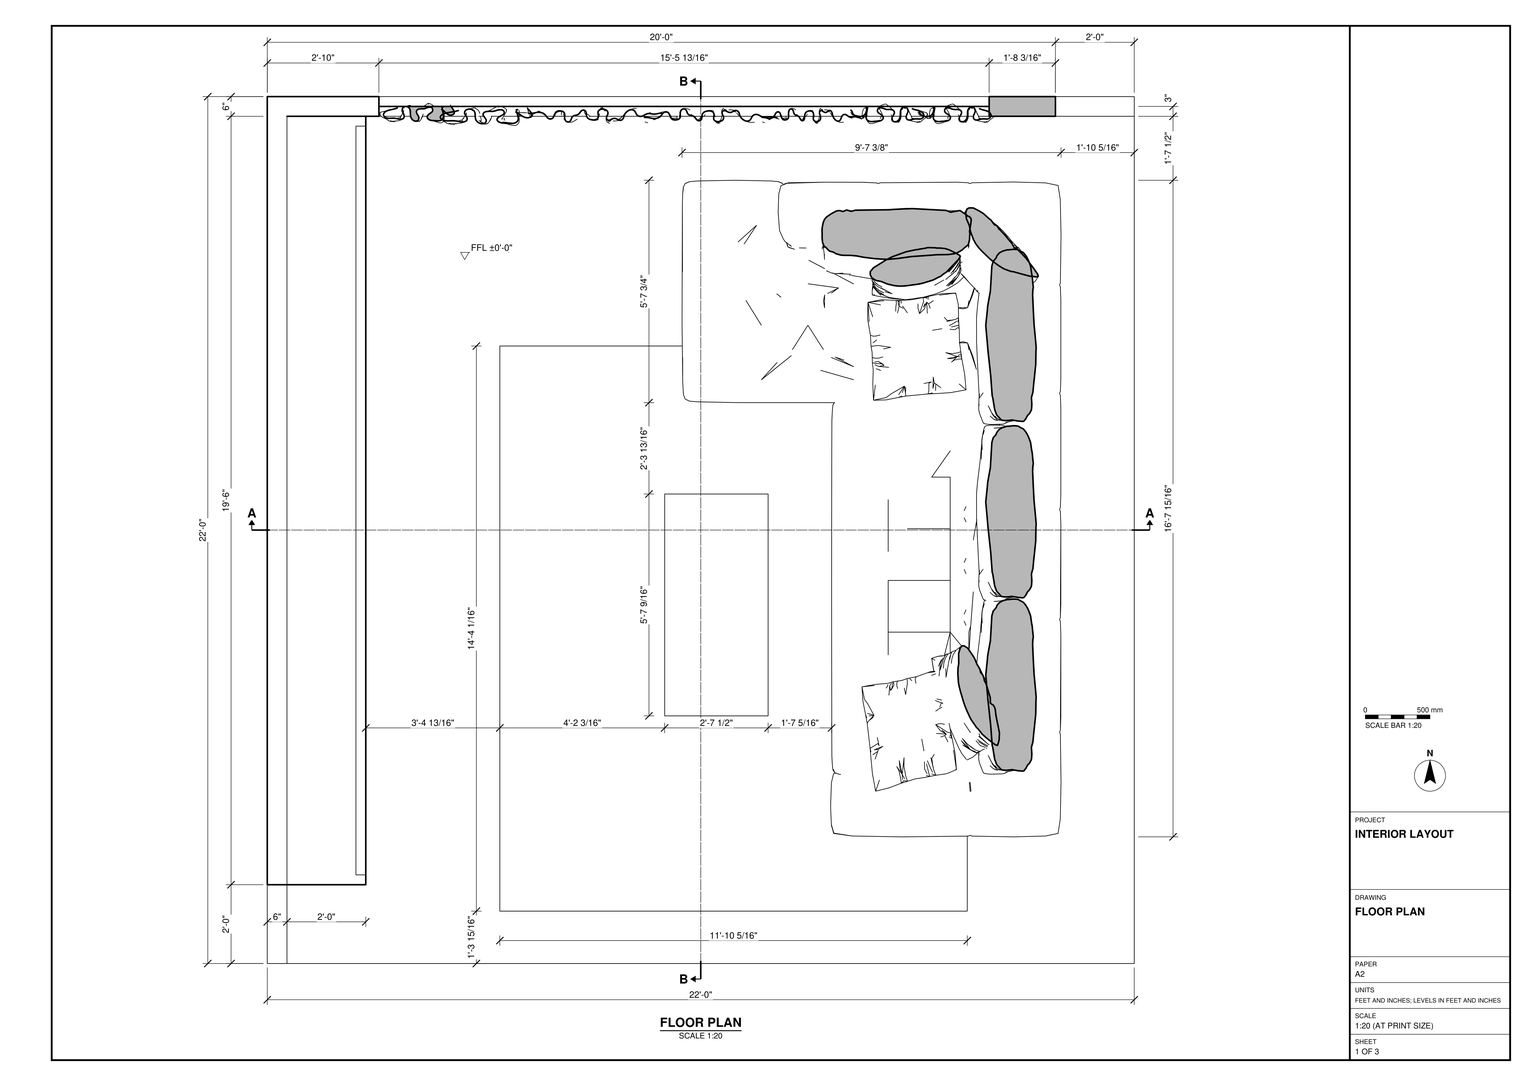
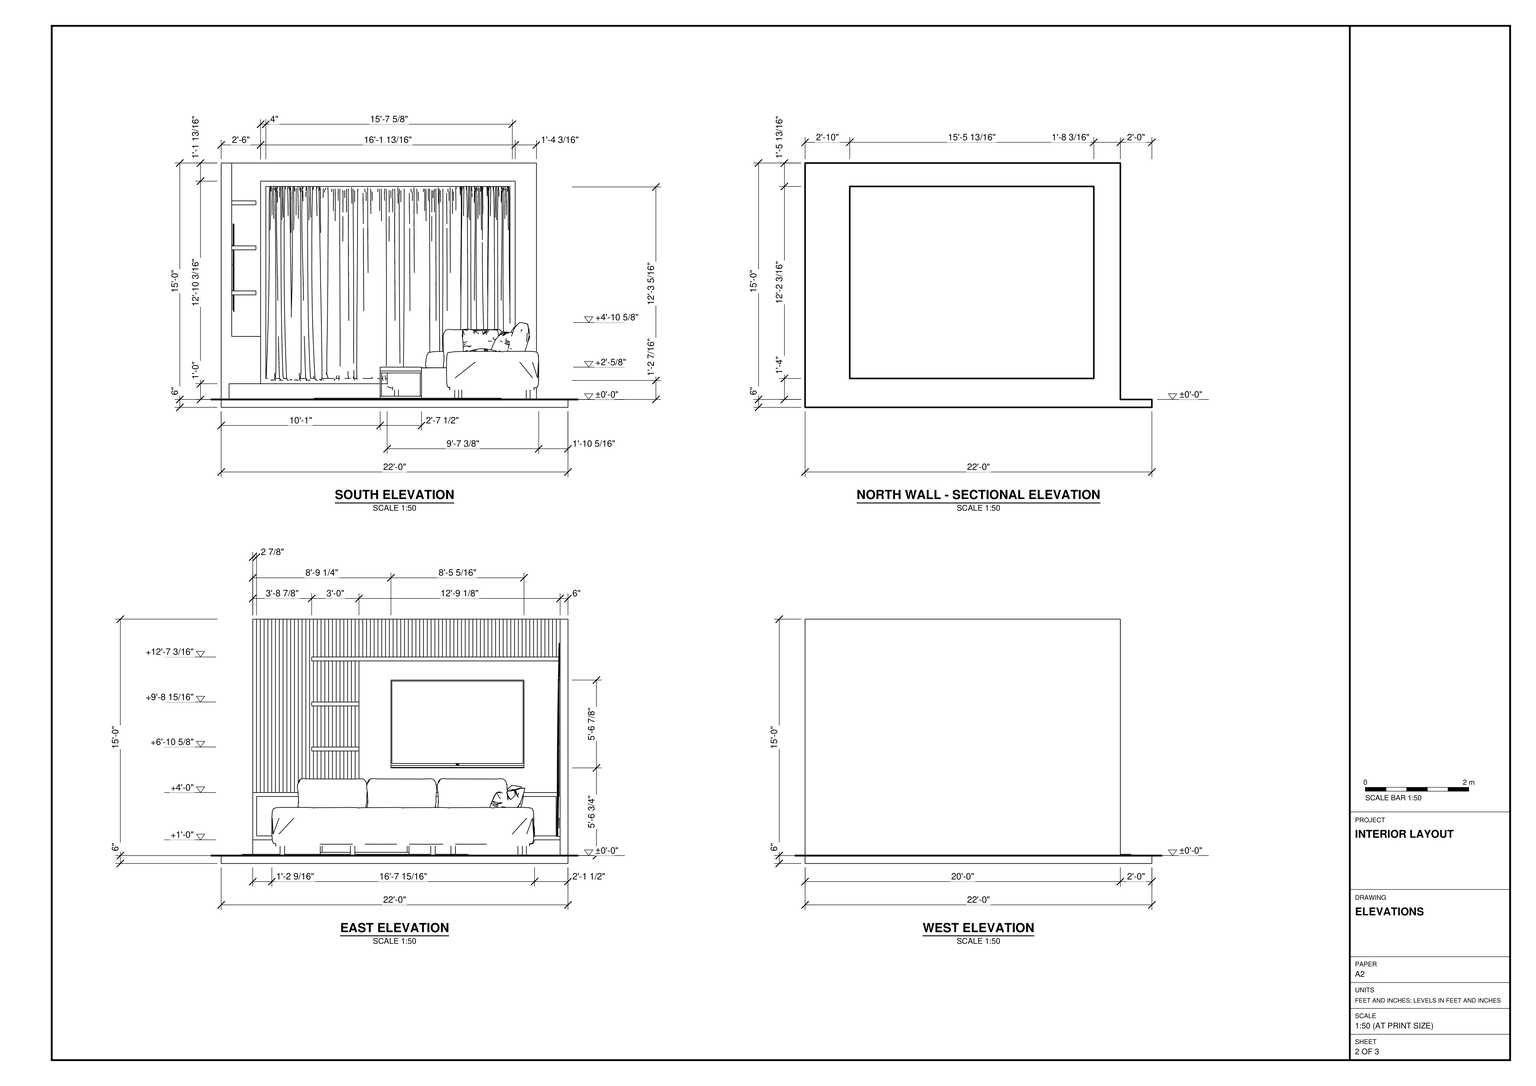
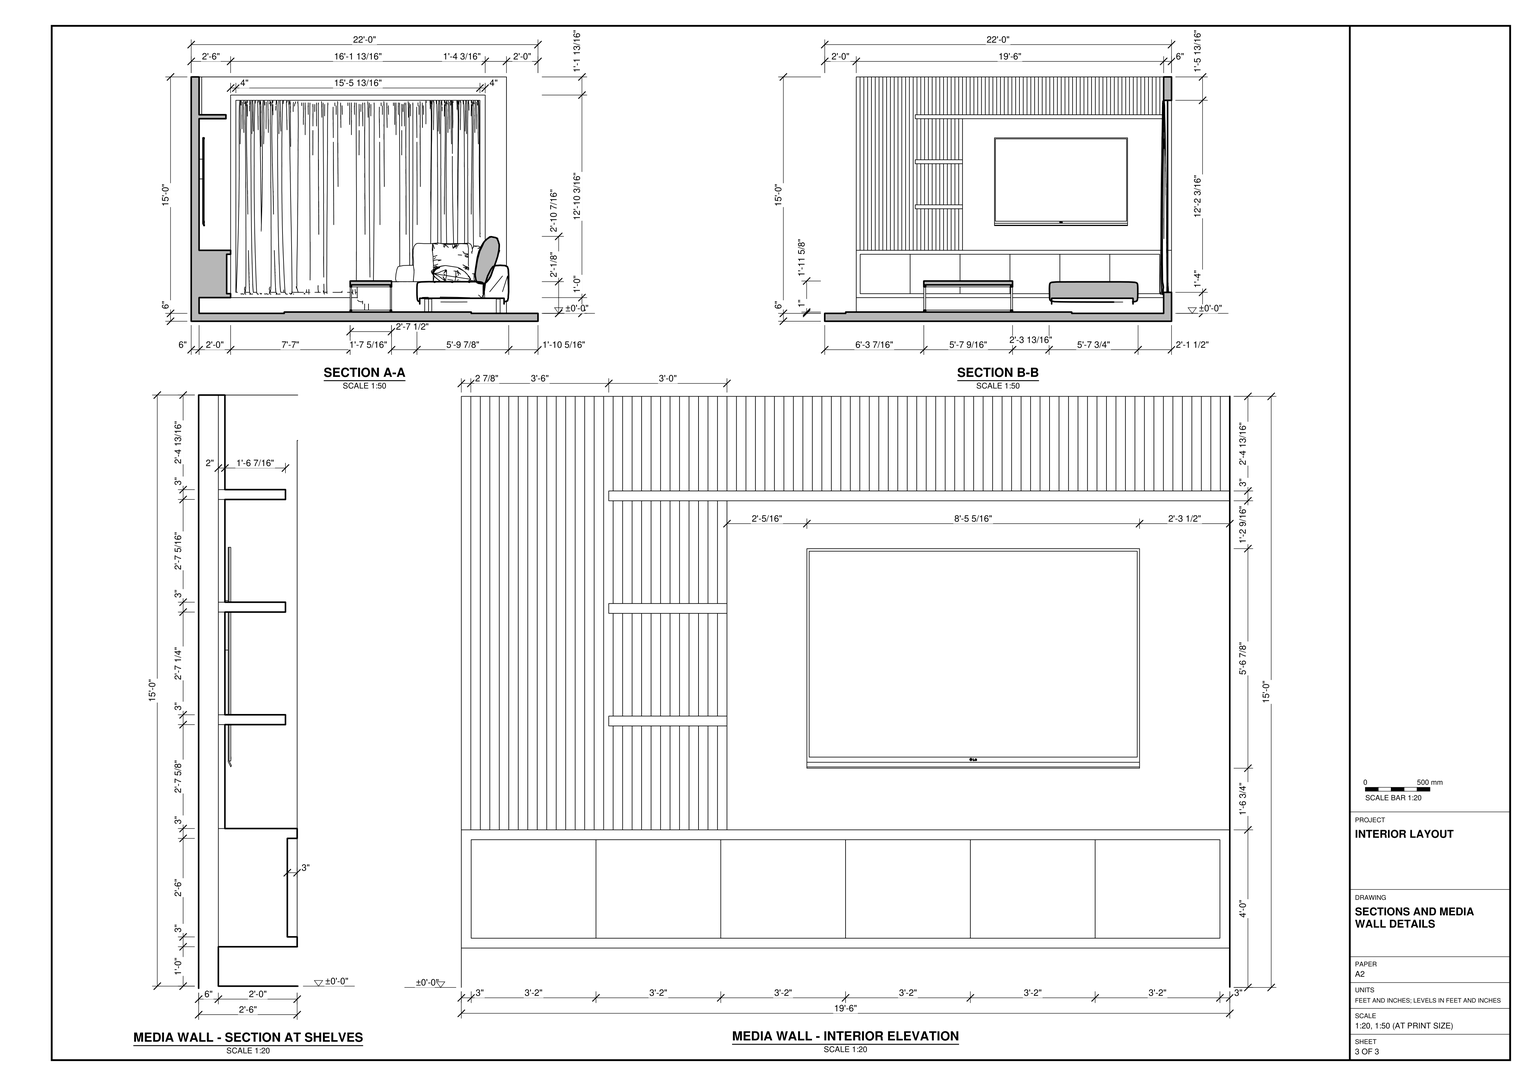
Build the living room in SketchUp from task_files/diagram_01.pdf. Work in feet and inches. The overall model is 22'-0" wide, 22'-0" deep and 15'-6" high. Set the finished floor at ±0'-0", with the 6" slab below it. Use the floor plan to place the 6" walls along the north and west sides, leaving the other sides open as drawn. Form the wide opening in the north wall, retaining the sill, head and unequal side returns. Hang the curtains across the opening.

Use the media wall elevation and shelf section to build the joinery on the inside face of the west wall. Include the raised cabinet with divided fronts, the vertical slats, the long upper shelf and the two shorter shelves beside the television. Place the sectional sofa opposite the television, with its long back on the east side and its chaise extending west at the north end. Set the low rectangular table between the sofa and cabinet, on the rug shown in plan. Decor and loose items, including the rug, cushions and television, may be any suitable library components.

Keep the walls, slab and each furniture or joinery piece in separate groups or components, and use components for repeated parts. Save one SketchUp model as output_files/living_room_with_a_built_in_media_wall.skp.

# SketchUp Ruby script. Lengths in inches.
U = 1.inch
M = Sketchup.active_model
def pt(a) = Geom::Point3d.new(a.map { |v| v * U })
def face(e, loops, mat)
  f = e.add_face(loops[0].map { |a| pt(a) })
  loops[1..].each { |l| e.add_face(l.map { |a| pt(a) }).erase! }
  f.material = f.back_material = mat if mat
  f
end
# faces: each face lists its corners as indices into pts; further lists are holes
def faces(e, pts, list, mat = nil) = list.each { |f| face(e, (f[0].is_a?(Array) ? f : [f]).map { |l| l.map { |i| pts[i] } }, mat) }
# xy, xz, yz: faces in a plane at the given z, y or x. An outline is a flat list of corners, or four numbers for a rectangle; further outlines are holes
def ring(l) = l.size == 4 ? [[l[0], l[1]], [l[2], l[1]], [l[2], l[3]], [l[0], l[3]]] : l.each_slice(2).to_a
def flat(e, list, mat, &to3) = list.each { |f| face(e, (f[0].is_a?(Array) ? f : [f]).map { |l| ring(l).map { |u, v| to3.(u, v) } }, mat) }
def xy(e, z, list, mat = nil) = flat(e, list, mat) { |x, y| [x, y, z] }
def xz(e, y, list, mat = nil) = flat(e, list, mat) { |x, z| [x, y, z] }
def yz(e, x, list, mat = nil) = flat(e, list, mat) { |y, z| [x, y, z] }
def lines(e, pts, list) = list.each { |a, b| e.add_line(pt(pts[a]), pt(pts[b])) }
# prism: a flat outline (further loops are holes) pulled along v
def prism(e, loops, v, mat = nil)
  f = face(e, loops, mat); d = Geom::Vector3d.new(v.map { |x| x * U })
  f.pushpull(f.normal.samedirection?(d) ? d.length : -d.length)
end
def box(e, o, s, mat = nil) = prism(e, [[o, [o[0] + s[0], o[1], o[2]], [o[0] + s[0], o[1] + s[1], o[2]], [o[0], o[1] + s[1], o[2]]]], [0, 0, s[2]], mat)
def at(x, y, z, deg = 0) = Geom::Transformation.translation(pt([x, y, z])) * Geom::Transformation.rotation(ORIGIN, Z_AXIS, deg.degrees)
def axes(o, x, y, z) = Geom::Transformation.new([*x, 0, *y, 0, *z, 0, *pt(o).to_a, 1])
def part(name) = M.definitions.add(name)
# library, detail: a bought-in or finely detailed component or shape, given as its bounding box
def library(name, o, s) = part(name).tap { |d| box(d.entities, o, s) }
def detail(e, o, s) = box(e.add_group.entities, o, s)
def put(e, d, t, mat = nil) = e.add_instance(d, t).tap { |i| i.material = mat if mat }
def group(e, t, mat = nil) = e.add_group.tap { |g| g.transformation = t; g.material = mat if mat }.entities
root = M.entities
M.materials.add("DefaultMaterial~1").color = [7, 7, 6]
M.materials.add("[0131_Silver]").color = [192, 192, 192]
M.materials.add("[0136_Charcoal]").color = [35, 35, 35]
M.materials.add("[Color_008]3").color = [29, 29, 29]
M.materials.add("[Formica Graystone]").color = [188, 184, 170]
M.materials.add("[Translucent Glass Blue]").color = [100, 149, 237]
M.materials["[Translucent Glass Blue]"].alpha = 0.5
c1 = library("TV (1)",[0,0,0],[57.09,0.98,33.46])
c2 = library("sofa (1)",[21.72,74.94,0],[120.18,81.27,34.35])
c3 = part("Group\#116")
box(c3.entities,[0,0,0],[0.98,0.98,11.8125])
c4 = part("center table rec")
g1 = group(c4.entities,at(39.79,0,0,90))
g2 = group(g1,at(0,0,0),"[Color_008]3")
put(g2,c3,at(0,-7.46,0.98))
g3 = group(g2,at(0,38.8,0.98))
box(g3,[0,0,0],[0.98,0.98,11.8125])
g4 = group(g2,at(30.51,38.8,0.98))
box(g4,[0,0,0],[0.98,0.98,11.8125])
put(g2,c3,at(30.51,-7.46,0.98))
g5 = group(g2,at(0,0,12.8))
prism(g5,[[[31.5,-7.46,0],[0,-7.46,0],[0,39.79,0],[31.5,39.79,0]],[[30.51,-6.47,0],[30.51,38.8,0],[0.98,38.8,0],[0.98,-6.47,0]]],[0,0,0.98])
g6 = group(g2,at(0,0,0))
prism(g6,[[[31.5,-7.46,0],[0,-7.46,0],[0,39.79,0],[31.5,39.79,0]],[[30.51,-6.47,0],[30.51,38.8,0],[0.98,38.8,0],[0.98,-6.47,0]]],[0,0,0.98])
g7 = group(g1,at(0,0,13.78))
xy(g7,0,[[0,-7.46,31.5,39.79]],"DefaultMaterial~1")
xy(g7,1.97,[[0.06,-7.4,0.08,-7.38,0.08,39.71,0.06,39.73],[0.06,-7.4,31.4375,-7.4,31.42,-7.38,0.08,-7.38],[31.4375,-7.4,31.4375,39.73,31.42,39.71,31.42,-7.38],[0.08,-7.38,31.42,39.71],[0.08,39.71,31.42,39.71,31.4375,39.73,0.06,39.73]],"DefaultMaterial~1")
xz(g7,-7.46,[[0,0,31.5,1.89]],"DefaultMaterial~1")
xz(g7,-7.45,[[0,1.91,31.49,1.91,31.49,1.93,0.01,1.93]],"DefaultMaterial~1")
xz(g7,39.78,[[0,1.91,0.01,1.93,31.49,1.93,31.49,1.91]],"DefaultMaterial~1")
xz(g7,39.79,[[0,0,31.5,1.89]],"DefaultMaterial~1")
yz(g7,0,[[-7.46,0,39.79,1.89],[-7.46,1.89,-7.45,1.91,39.78,1.91,39.79,1.89]],"DefaultMaterial~1")
yz(g7,31.49,[[-7.45,1.91,39.78,1.93]],"DefaultMaterial~1")
yz(g7,31.5,[[-7.46,0,39.79,1.89]],"DefaultMaterial~1")
p = [[0,-7.46,1.89],[31.5,-7.46,1.89],[31.49,-7.45,1.91],[0,-7.45,1.91],[0,39.78,1.91],[0.01,-7.45,1.93],
  [0.01,39.78,1.93],[31.5,39.79,1.89],[31.49,39.78,1.91],[0.02,39.76,1.95],[0.02,-7.43,1.95],[0.04,-7.42,1.96],
  [0.04,39.75,1.96],[31.47,-7.43,1.95],[31.46,-7.42,1.96],[31.49,-7.45,1.93],[31.49,39.78,1.93],[31.47,39.76,1.95],
  [31.46,39.75,1.96],[0,39.79,1.89],[31.4375,-7.4,1.97],[0.06,-7.4,1.97],[0.06,39.73,1.97],[31.4375,39.73,1.97]]
faces(g7,p,[[0,1,2,3],[4,3,5,6],[1,7,8,2],[9,10,11,12],[6,5,10,9],[10,13,14,11],[5,15,13,10],[15,16,17,13],
  [13,17,18,14],[17,9,12,18],[7,19,4,8],[16,6,9,17],[11,14,20,21],[12,11,21,22],[14,18,23,20],[18,12,22,23]],"DefaultMaterial~1")
c5 = part("CENTER+TABLE+REC2")
put(c5.entities,c4,at(0,0,0))
c6 = library("Group5_1",[-7.56,-50.83,0.1],[6.91,117.83,114.21])
xy(root,0,[[0,0,264,264]])
xy(root,6,[[0,0,6,24],[240,258,264,264]])
xy(root,6,[[[6,0,264,258],[70.82,15.96,213.16,188.04]]],"[0131_Silver]")
xy(root,7,[[70.82,15.96,213.16,188.04]],"[Formica Graystone]")
xy(root,18,[[6,24,30,258]])
xy(root,21,[[27,27,30,255]],"[0136_Charcoal]")
xy(root,22,[[34,258,219.8125,261],[34,261,219.8125,264]])
xy(root,51,[[27,27,30,255]],"[0136_Charcoal]")
xy(root,54,[[8,24,30,24,30,258,6,258,6,102,8,102,8,99.11,6,99.11,6,96.22,8,96.22,8,93.33,6,93.33,6,90.44,8,90.44,8,87.56,6,87.56,6,84.67,8,84.67,8,81.78,6,81.78,6,78.89,8,78.89,8,76,6,76,6,73.11,8,73.11,8,70.22,6,70.22,6,67.33,8,67.33,8,64.44,6,64.44,6,61.56,8,61.56,8,58.67,6,58.67,6,55.78,8,55.78,8,52.89,6,52.89,6,50,8,50,8,47.11,6,47.11,6,44.22,8,44.22,8,41.33,6,41.33,6,38.44,8,38.44,8,35.56,6,35.56,6,32.67,8,32.67,8,29.78,6,29.78,6,26.89,8,26.89]],"[0136_Charcoal]")
xy(root,85.64,[[6,68.89,6,70.22,8,70.22,8,73.11,6,73.11,6,76,8,76,8,78.89,6,78.89,6,81.78,8,81.78,8,84.67,6,84.67,6,87.56,8,87.56,8,90.44,6,90.44,6,93.33,8,93.33,8,96.22,6,96.22,6,99.11,8,99.11,8,102,6,102,6,104.89,26.4375,104.89,26.4375,68.89]],"[0136_Charcoal]")
xy(root,88.64,[[6,68.89,26.4375,68.89,26.4375,104.89,6,104.89,6,102,8,102,8,99.11,6,99.11,6,96.22,8,96.22,8,93.33,6,93.33,6,90.44,8,90.44,8,87.56,6,87.56,6,84.67,8,84.67,8,81.78,6,81.78,6,78.89,8,78.89,8,76,6,76,6,73.11,8,73.11,8,70.22,6,70.22]],"[0136_Charcoal]")
xy(root,108.34,[[6,164.33,9,183.15]])
xy(root,119.92,[[6,68.89,6,70.22,8,70.22,8,73.11,6,73.11,6,76,8,76,8,78.89,6,78.89,6,81.78,8,81.78,8,84.67,6,84.67,6,87.56,8,87.56,8,90.44,6,90.44,6,93.33,8,93.33,8,96.22,6,96.22,6,99.11,8,99.11,8,102,6,102,6,104.89,26.4375,104.89,26.4375,68.89]],"[0136_Charcoal]")
xy(root,122.92,[[6,68.89,26.4375,68.89,26.4375,104.89,6,104.89,6,102,8,102,8,99.11,6,99.11,6,96.22,8,96.22,8,93.33,6,93.33,6,90.44,8,90.44,8,87.56,6,87.56,6,84.67,8,84.67,8,81.78,6,81.78,6,78.89,8,78.89,8,76,6,76,6,73.11,8,73.11,8,70.22,6,70.22]],"[0136_Charcoal]")
xy(root,123.41,[[6,164.33,9,183.15]])
xy(root,154.2,[[6,68.89,6,70.22,8,70.22,8,73.11,6,73.11,6,76,8,76,8,78.89,6,78.89,6,81.78,8,81.78,8,84.67,6,84.67,6,87.56,8,87.56,8,90.44,6,90.44,6,93.33,8,93.33,8,96.22,6,96.22,6,99.11,8,99.11,8,102,6,102,6,258,26.4375,258,26.4375,68.89]],"[0136_Charcoal]")
xy(root,157.2,[[6,68.89,26.4375,68.89,26.4375,258,8,258,8,255.11,6,255.11,6,252.22,8,252.22,8,249.33,6,249.33,6,246.44,8,246.44,8,243.56,6,243.56,6,240.67,8,240.67,8,237.78,6,237.78,6,234.89,8,234.89,8,232,6,232,6,229.11,8,229.11,8,226.22,6,226.22,6,223.33,8,223.33,8,220.44,6,220.44,6,217.56,8,217.56,8,214.67,6,214.67,6,211.78,8,211.78,8,208.89,6,208.89,6,206,8,206,8,203.11,6,203.11,6,200.22,8,200.22,8,197.33,6,197.33,6,194.44,8,194.44,8,191.56,6,191.56,6,188.67,8,188.67,8,185.78,6,185.78,6,182.89,8,182.89,8,180,6,180,6,177.11,8,177.11,8,174.22,6,174.22,6,171.33,8,171.33,8,168.44,6,168.44,6,165.56,8,165.56,8,162.67,6,162.67,6,159.78,8,159.78,8,156.89,6,156.89,6,154,8,154,8,151.11,6,151.11,6,148.22,8,148.22,8,145.33,6,145.33,6,142.44,8,142.44,8,139.56,6,139.56,6,136.67,8,136.67,8,133.78,6,133.78,6,130.89,8,130.89,8,128,6,128,6,125.11,8,125.11,8,122.22,6,122.22,6,119.33,8,119.33,8,116.44,6,116.44,6,113.56,8,113.56,8,110.67,6,110.67,6,107.78,8,107.78,8,104.89,6,104.89,6,102,8,102,8,99.11,6,99.11,6,96.22,8,96.22,8,93.33,6,93.33,6,90.44,8,90.44,8,87.56,6,87.56,6,84.67,8,84.67,8,81.78,6,81.78,6,78.89,8,78.89,8,76,6,76,6,73.11,8,73.11,8,70.22,6,70.22]],"[0136_Charcoal]")
xy(root,168.1875,[[34,258,219.8125,261],[34,261,219.8125,264]])
xy(root,186,[[0,24,8,24,8,26.89,6,26.89,6,29.78,8,29.78,8,32.67,6,32.67,6,35.56,8,35.56,8,38.44,6,38.44,6,41.33,8,41.33,8,44.22,6,44.22,6,47.11,8,47.11,8,50,6,50,6,52.89,8,52.89,8,55.78,6,55.78,6,58.67,8,58.67,8,61.56,6,61.56,6,64.44,8,64.44,8,67.33,6,67.33,6,70.22,8,70.22,8,73.11,6,73.11,6,76,8,76,8,78.89,6,78.89,6,81.78,8,81.78,8,84.67,6,84.67,6,87.56,8,87.56,8,90.44,6,90.44,6,93.33,8,93.33,8,96.22,6,96.22,6,99.11,8,99.11,8,102,6,102,6,104.89,8,104.89,8,107.78,6,107.78,6,110.67,8,110.67,8,113.56,6,113.56,6,116.44,8,116.44,8,119.33,6,119.33,6,122.22,8,122.22,8,125.11,6,125.11,6,128,8,128,8,130.89,6,130.89,6,133.78,8,133.78,8,136.67,6,136.67,6,139.56,8,139.56,8,142.44,6,142.44,6,145.33,8,145.33,8,148.22,6,148.22,6,151.11,8,151.11,8,154,6,154,6,156.89,8,156.89,8,159.78,6,159.78,6,162.67,8,162.67,8,165.56,6,165.56,6,168.44,8,168.44,8,171.33,6,171.33,6,174.22,8,174.22,8,177.11,6,177.11,6,180,8,180,8,182.89,6,182.89,6,185.78,8,185.78,8,188.67,6,188.67,6,191.56,8,191.56,8,194.44,6,194.44,6,197.33,8,197.33,8,200.22,6,200.22,6,203.11,8,203.11,8,206,6,206,6,208.89,8,208.89,8,211.78,6,211.78,6,214.67,8,214.67,8,217.56,6,217.56,6,220.44,8,220.44,8,223.33,6,223.33,6,226.22,8,226.22,8,229.11,6,229.11,6,232,8,232,8,234.89,6,234.89,6,237.78,8,237.78,8,240.67,6,240.67,6,243.56,8,243.56,8,246.44,6,246.44,6,249.33,8,249.33,8,252.22,6,252.22,6,255.11,8,255.11,8,258,6,258,6,264,0,264],[6,258,240,264]])
xz(root,0,[[0,0,264,6]])
xz(root,15.96,[[70.82,6,213.16,7]],"[Formica Graystone]")
xz(root,24,[[0,6,6,6,6,18,30,18,30,54,8,54,8,186,0,186]],"[0136_Charcoal]")
xz(root,26.89,[[6,54,8,186]],"[0136_Charcoal]")
xz(root,27,[[27,21,30,51]],"[0136_Charcoal]")
xz(root,29.78,[[6,54,8,186]],"[0136_Charcoal]")
xz(root,32.67,[[6,54,8,186]],"[0136_Charcoal]")
xz(root,35.56,[[6,54,8,186]],"[0136_Charcoal]")
xz(root,38.44,[[6,54,8,186]],"[0136_Charcoal]")
xz(root,41.33,[[6,54,8,186]],"[0136_Charcoal]")
xz(root,44.22,[[6,54,8,186]],"[0136_Charcoal]")
xz(root,47.11,[[6,54,8,186]],"[0136_Charcoal]")
xz(root,50,[[6,54,8,186]],"[0136_Charcoal]")
xz(root,52.89,[[6,54,8,186]],"[0136_Charcoal]")
xz(root,55.78,[[6,54,8,186]],"[0136_Charcoal]")
xz(root,58.67,[[6,54,8,186]],"[0136_Charcoal]")
xz(root,61.56,[[6,54,8,186]],"[0136_Charcoal]")
xz(root,64.44,[[6,54,8,186]],"[0136_Charcoal]")
xz(root,67.33,[[6,54,8,186]],"[0136_Charcoal]")
xz(root,68.89,[[6,85.64,26.4375,88.64],[6,119.92,26.4375,122.92],[6,154.2,26.4375,157.2]],"[0136_Charcoal]")
xz(root,70.22,[[6,54,8,85.64],[6,88.64,8,119.92],[6,122.92,8,154.2],[6,157.2,8,186]],"[0136_Charcoal]")
xz(root,73.11,[[6,54,8,85.64],[6,88.64,8,119.92],[6,122.92,8,154.2],[6,157.2,8,186]],"[0136_Charcoal]")
xz(root,76,[[6,54,8,85.64],[6,88.64,8,119.92],[6,122.92,8,154.2],[6,157.2,8,186]],"[0136_Charcoal]")
xz(root,78.89,[[6,54,8,85.64],[6,88.64,8,119.92],[6,122.92,8,154.2],[6,157.2,8,186]],"[0136_Charcoal]")
xz(root,81.78,[[6,54,8,85.64],[6,88.64,8,119.92],[6,122.92,8,154.2],[6,157.2,8,186]],"[0136_Charcoal]")
xz(root,84.67,[[6,54,8,85.64],[6,88.64,8,119.92],[6,122.92,8,154.2],[6,157.2,8,186]],"[0136_Charcoal]")
xz(root,87.56,[[6,54,8,85.64],[6,88.64,8,119.92],[6,122.92,8,154.2],[6,157.2,8,186]],"[0136_Charcoal]")
xz(root,90.44,[[6,54,8,85.64],[6,88.64,8,119.92],[6,122.92,8,154.2],[6,157.2,8,186]],"[0136_Charcoal]")
xz(root,93.33,[[6,54,8,85.64],[6,88.64,8,119.92],[6,122.92,8,154.2],[6,157.2,8,186]],"[0136_Charcoal]")
xz(root,96.22,[[6,54,8,85.64],[6,88.64,8,119.92],[6,122.92,8,154.2],[6,157.2,8,186]],"[0136_Charcoal]")
xz(root,99.11,[[6,54,8,85.64],[6,88.64,8,119.92],[6,122.92,8,154.2],[6,157.2,8,186]],"[0136_Charcoal]")
xz(root,102,[[6,54,8,85.64],[6,88.64,8,119.92],[6,122.92,8,154.2],[6,157.2,8,186]],"[0136_Charcoal]")
xz(root,104.89,[[6,85.64,26.4375,88.64],[6,119.92,26.4375,122.92],[6,157.2,8,186]],"[0136_Charcoal]")
xz(root,107.78,[[6,157.2,8,186]],"[0136_Charcoal]")
xz(root,110.67,[[6,157.2,8,186]],"[0136_Charcoal]")
xz(root,113.56,[[6,157.2,8,186]],"[0136_Charcoal]")
xz(root,116.44,[[6,157.2,8,186]],"[0136_Charcoal]")
xz(root,119.33,[[6,157.2,8,186]],"[0136_Charcoal]")
xz(root,122.22,[[6,157.2,8,186]],"[0136_Charcoal]")
xz(root,125.11,[[6,157.2,8,186]],"[0136_Charcoal]")
xz(root,128,[[6,157.2,8,186]],"[0136_Charcoal]")
xz(root,130.89,[[6,157.2,8,186]],"[0136_Charcoal]")
xz(root,133.78,[[6,157.2,8,186]],"[0136_Charcoal]")
xz(root,136.67,[[6,157.2,8,186]],"[0136_Charcoal]")
xz(root,139.56,[[6,157.2,8,186]],"[0136_Charcoal]")
xz(root,142.44,[[6,157.2,8,186]],"[0136_Charcoal]")
xz(root,145.33,[[6,157.2,8,186]],"[0136_Charcoal]")
xz(root,148.22,[[6,157.2,8,186]],"[0136_Charcoal]")
xz(root,151.11,[[6,157.2,8,186]],"[0136_Charcoal]")
xz(root,154,[[6,157.2,8,186]],"[0136_Charcoal]")
xz(root,156.89,[[6,157.2,8,186]],"[0136_Charcoal]")
xz(root,159.78,[[6,157.2,8,186]],"[0136_Charcoal]")
xz(root,162.67,[[6,157.2,8,186]],"[0136_Charcoal]")
xz(root,164.33,[[6,108.34,9,123.41]])
xz(root,165.56,[[6,157.2,8,186]],"[0136_Charcoal]")
xz(root,168.44,[[6,157.2,8,186]],"[0136_Charcoal]")
xz(root,171.33,[[6,157.2,8,186]],"[0136_Charcoal]")
xz(root,174.22,[[6,157.2,8,186]],"[0136_Charcoal]")
xz(root,177.11,[[6,157.2,8,186]],"[0136_Charcoal]")
xz(root,180,[[6,157.2,8,186]],"[0136_Charcoal]")
xz(root,182.89,[[6,157.2,8,186]],"[0136_Charcoal]")
xz(root,183.15,[[6,108.34,9,123.41]])
xz(root,185.78,[[6,157.2,8,186]],"[0136_Charcoal]")
xz(root,188.04,[[70.82,6,213.16,7]],"[Formica Graystone]")
xz(root,188.67,[[6,157.2,8,186]],"[0136_Charcoal]")
xz(root,191.56,[[6,157.2,8,186]],"[0136_Charcoal]")
xz(root,194.44,[[6,157.2,8,186]],"[0136_Charcoal]")
xz(root,197.33,[[6,157.2,8,186]],"[0136_Charcoal]")
xz(root,200.22,[[6,157.2,8,186]],"[0136_Charcoal]")
xz(root,203.11,[[6,157.2,8,186]],"[0136_Charcoal]")
xz(root,206,[[6,157.2,8,186]],"[0136_Charcoal]")
xz(root,208.89,[[6,157.2,8,186]],"[0136_Charcoal]")
xz(root,211.78,[[6,157.2,8,186]],"[0136_Charcoal]")
xz(root,214.67,[[6,157.2,8,186]],"[0136_Charcoal]")
xz(root,217.56,[[6,157.2,8,186]],"[0136_Charcoal]")
xz(root,220.44,[[6,157.2,8,186]],"[0136_Charcoal]")
xz(root,223.33,[[6,157.2,8,186]],"[0136_Charcoal]")
xz(root,226.22,[[6,157.2,8,186]],"[0136_Charcoal]")
xz(root,229.11,[[6,157.2,8,186]],"[0136_Charcoal]")
xz(root,232,[[6,157.2,8,186]],"[0136_Charcoal]")
xz(root,234.89,[[6,157.2,8,186]],"[0136_Charcoal]")
xz(root,237.78,[[6,157.2,8,186]],"[0136_Charcoal]")
xz(root,240.67,[[6,157.2,8,186]],"[0136_Charcoal]")
xz(root,243.56,[[6,157.2,8,186]],"[0136_Charcoal]")
xz(root,246.44,[[6,157.2,8,186]],"[0136_Charcoal]")
xz(root,249.33,[[6,157.2,8,186]],"[0136_Charcoal]")
xz(root,252.22,[[6,157.2,8,186]],"[0136_Charcoal]")
xz(root,255,[[27,21,30,51]],"[0136_Charcoal]")
xz(root,255.11,[[6,157.2,8,186]],"[0136_Charcoal]")
xz(root,258,[[6,18,30,54],[6,154.2,26.4375,157.2],[6,157.2,8,186]])
xz(root,258,[[[6,6,240,6,240,186,8,186,8,157.2,26.4375,157.2,26.4375,154.2,6,154.2],[30,18,223.8125,172.1875]],[[30,18,223.8125,172.1875],[34,22,219.8125,168.1875]]],"[0131_Silver]")
xz(root,261,[[34,22,219.8125,168.1875]],"[Translucent Glass Blue]")
xz(root,264,[[[0,0,0,186,240,186,240,6,264,6,264,0],[34,22,219.8125,168.1875]]])
yz(root,0,[[0,0,0,6,24,6,24,186,264,186,264,0]])
yz(root,6,[[[104.89,54,258,154.2],[164.33,108.34,183.15,123.41]]],"[0131_Silver]")
yz(root,6,[[24,6,258,18],[26.89,54,29.78,186],[32.67,54,35.56,186],[38.44,54,41.33,186],[44.22,54,47.11,186],
  [50,54,52.89,186],[55.78,54,58.67,186],[61.56,54,64.44,186],[67.33,54,70.22,54,70.22,85.64,68.89,85.64,68.89,88.64,70.22,88.64,70.22,119.92,68.89,119.92,68.89,122.92,70.22,122.92,70.22,154.2,68.89,154.2,68.89,157.2,70.22,157.2,70.22,186,67.33,186],[73.11,54,76,85.64],
  [78.89,54,81.78,85.64],[84.67,54,87.56,85.64],[90.44,54,93.33,85.64],[96.22,54,99.11,85.64],[102,54,104.89,85.64],
  [73.11,88.64,76,119.92],[78.89,88.64,81.78,119.92],[84.67,88.64,87.56,119.92],[90.44,88.64,93.33,119.92],[96.22,88.64,99.11,119.92],
  [102,88.64,104.89,119.92],[73.11,122.92,76,154.2],[78.89,122.92,81.78,154.2],[84.67,122.92,87.56,154.2],[90.44,122.92,93.33,154.2],
  [96.22,122.92,99.11,154.2],[102,122.92,104.89,154.2],[73.11,157.2,76,186],[78.89,157.2,81.78,186],[84.67,157.2,87.56,186],
  [90.44,157.2,93.33,186],[96.22,157.2,99.11,186],[102,157.2,104.89,186],[107.78,157.2,110.67,186],[113.56,157.2,116.44,186],
  [119.33,157.2,122.22,186],[125.11,157.2,128,186],[130.89,157.2,133.78,186],[136.67,157.2,139.56,186],[142.44,157.2,145.33,186],
  [148.22,157.2,151.11,186],[154,157.2,156.89,186],[159.78,157.2,162.67,186],[165.56,157.2,168.44,186],[171.33,157.2,174.22,186],
  [177.11,157.2,180,186],[182.89,157.2,185.78,186],[188.67,157.2,191.56,186],[194.44,157.2,197.33,186],[200.22,157.2,203.11,186],
  [206,157.2,208.89,186],[211.78,157.2,214.67,186],[217.56,157.2,220.44,186],[223.33,157.2,226.22,186],[229.11,157.2,232,186],
  [234.89,157.2,237.78,186],[240.67,157.2,243.56,186],[246.44,157.2,249.33,186],[252.22,157.2,255.11,186]],"[0136_Charcoal]")
yz(root,8,[[24,54,26.89,186],[29.78,54,32.67,186],[35.56,54,38.44,186],[41.33,54,44.22,186],[47.11,54,50,186],
  [52.89,54,55.78,186],[58.67,54,61.56,186],[64.44,54,67.33,186],[70.22,54,73.11,85.64],[76,54,78.89,85.64],
  [81.78,54,84.67,85.64],[87.56,54,90.44,85.64],[93.33,54,96.22,85.64],[99.11,54,102,85.64],[70.22,88.64,73.11,119.92],
  [76,88.64,78.89,119.92],[81.78,88.64,84.67,119.92],[87.56,88.64,90.44,119.92],[93.33,88.64,96.22,119.92],[99.11,88.64,102,119.92],
  [70.22,122.92,73.11,154.2],[76,122.92,78.89,154.2],[81.78,122.92,84.67,154.2],[87.56,122.92,90.44,154.2],[93.33,122.92,96.22,154.2],
  [99.11,122.92,102,154.2],[70.22,157.2,73.11,186],[76,157.2,78.89,186],[81.78,157.2,84.67,186],[87.56,157.2,90.44,186],
  [93.33,157.2,96.22,186],[99.11,157.2,102,186],[104.89,157.2,107.78,186],[110.67,157.2,113.56,186],[116.44,157.2,119.33,186],
  [122.22,157.2,125.11,186],[128,157.2,130.89,186],[133.78,157.2,136.67,186],[139.56,157.2,142.44,186],[145.33,157.2,148.22,186],
  [151.11,157.2,154,186],[156.89,157.2,159.78,186],[162.67,157.2,165.56,186],[168.44,157.2,171.33,186],[174.22,157.2,177.11,186],
  [180,157.2,182.89,186],[185.78,157.2,188.67,186],[191.56,157.2,194.44,186],[197.33,157.2,200.22,186],[203.11,157.2,206,186],
  [208.89,157.2,211.78,186],[214.67,157.2,217.56,186],[220.44,157.2,223.33,186],[226.22,157.2,229.11,186],[232,157.2,234.89,186],
  [237.78,157.2,240.67,186],[243.56,157.2,246.44,186],[249.33,157.2,252.22,186],[255.11,157.2,258,186]],"[0136_Charcoal]")
yz(root,9,[[164.33,108.34,183.15,123.41]])
yz(root,26.4375,[[68.89,85.64,104.89,88.64],[68.89,119.92,104.89,122.92],[68.89,154.2,258,157.2]],"[0136_Charcoal]")
yz(root,27,[[27,21,65,51],[65,21,103,51],[103,21,141,51],[141,21,179,51],[179,21,217,51],
  [217,21,255,51]],"[0131_Silver]")
yz(root,30,[[[24,18,258,54],[27,21,255,51]]],"[0136_Charcoal]")
yz(root,34,[[258,22,261,168.1875],[261,22,264,54],[261,54,264,168.1875]])
yz(root,70.82,[[15.96,6,188.04,7]],"[Formica Graystone]")
yz(root,213.16,[[15.96,6,188.04,7]],"[Formica Graystone]")
yz(root,219.8125,[[258,22,261,168.1875],[261,22,264,168.1875]])
yz(root,240,[[258,6,264,186]])
yz(root,264,[[0,0,264,6]])
put(root,c1,axes([9.98,129.22,72.77],[0,1.7744,0],[-1,0,0],[0,0,1.998]),"[0136_Charcoal]")
put(root,c2,axes([19.88,274.67,6],[0,-1.6638,0],[1.42,0,0],[0,0,1.7061]))
put(root,c5,axes([152.51,75.42,7],[0,1.43,0],[-1,0,0],[0,0,1.5]))
put(root,c6,axes([114.9375,254.55,20.32],[0,-1,0],[1.59229,0,0],[0,0,1.29]))
